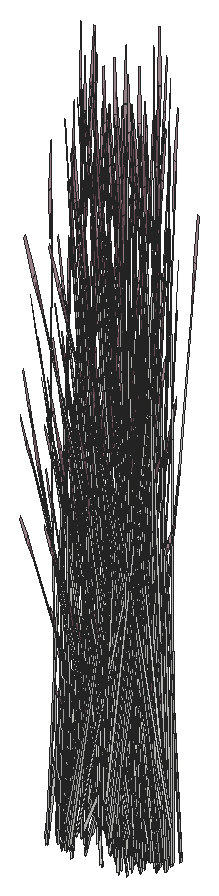
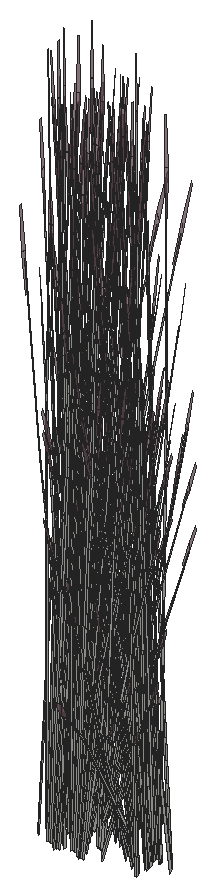
# SketchUp Ruby script. Lengths in inches.
U = 1.inch
M = Sketchup.active_model
def pt(a) = Geom::Point3d.new(a.map { |v| v * U })
def face(e, loops, mat)
  f = e.add_face(loops[0].map { |a| pt(a) })
  loops[1..].each { |l| e.add_face(l.map { |a| pt(a) }).erase! }
  f.material = f.back_material = mat if mat
  f
end
# faces: each face lists its corners as indices into pts; further lists are holes
def faces(e, pts, list, mat = nil) = list.each { |f| face(e, (f[0].is_a?(Array) ? f : [f]).map { |l| l.map { |i| pts[i] } }, mat) }
# xy, xz, yz: faces in a plane at the given z, y or x. An outline is a flat list of corners, or four numbers for a rectangle; further outlines are holes
def ring(l) = l.size == 4 ? [[l[0], l[1]], [l[2], l[1]], [l[2], l[3]], [l[0], l[3]]] : l.each_slice(2).to_a
def flat(e, list, mat, &to3) = list.each { |f| face(e, (f[0].is_a?(Array) ? f : [f]).map { |l| ring(l).map { |u, v| to3.(u, v) } }, mat) }
def xy(e, z, list, mat = nil) = flat(e, list, mat) { |x, y| [x, y, z] }
def xz(e, y, list, mat = nil) = flat(e, list, mat) { |x, z| [x, y, z] }
def yz(e, x, list, mat = nil) = flat(e, list, mat) { |y, z| [x, y, z] }
def lines(e, pts, list) = list.each { |a, b| e.add_line(pt(pts[a]), pt(pts[b])) }
# prism: a flat outline (further loops are holes) pulled along v
def prism(e, loops, v, mat = nil)
  f = face(e, loops, mat); d = Geom::Vector3d.new(v.map { |x| x * U })
  f.pushpull(f.normal.samedirection?(d) ? d.length : -d.length)
end
def box(e, o, s, mat = nil) = prism(e, [[o, [o[0] + s[0], o[1], o[2]], [o[0] + s[0], o[1] + s[1], o[2]], [o[0], o[1] + s[1], o[2]]]], [0, 0, s[2]], mat)
def at(x, y, z, deg = 0) = Geom::Transformation.translation(pt([x, y, z])) * Geom::Transformation.rotation(ORIGIN, Z_AXIS, deg.degrees)
def axes(o, x, y, z) = Geom::Transformation.new([*x, 0, *y, 0, *z, 0, *pt(o).to_a, 1])
def part(name) = M.definitions.add(name)
# library, detail: a bought-in or finely detailed component or shape, given as its bounding box
def library(name, o, s) = part(name).tap { |d| box(d.entities, o, s) }
def detail(e, o, s) = box(e.add_group.entities, o, s)
def put(e, d, t, mat = nil) = e.add_instance(d, t).tap { |i| i.material = mat if mat }
def group(e, t, mat = nil) = e.add_group.tap { |g| g.transformation = t; g.material = mat if mat }.entities
root = M.entities
M.materials.add("LightPink_Translucent").color = [144, 107, 117]
M.materials["LightPink_Translucent"].alpha = 0.75
c1 = part("blade")
p = [[2.15,0.21,22],[0,0.17,0],[0.09,0.45,0],[2.18,0.31,22],[2.29,0.31,22],[0.38,0.45,0],
  [2.48,0.24,33],[2.49,0.24,33],[2.48,0.22,33]]
faces(c1.entities,p,[[0,1,2,3],[4,5,2,3],[6,3,4,7],[8,0,3,6]])
c2 = part("seeds")
p = [[0.3,-0.1,1.38],[-0.01,-0.03,1.59],[-0.01,-0.03,0.03],[0.14,-0.07,-0.07],[0.29,-0.03,3],[0.15,0.01,3.11]]
faces(c2.entities,p,[[0,1,2,3],[1,0,4,5]],"LightPink_Translucent")
c3 = part("blade with seeds")
put(c3.entities,c1,at(0,0,0))
put(c3.entities,c2,axes([2.4,0.25,30.99],[1.5799,-0.05474,1.17369],[-0.12525,1.92788,0.29478],[-0.07173,-0.02425,1.56792]))
put(root,c3,axes([350.21,661.74,620.36],[-0.29264,0.42323,0.45755],[-0.34767,-0.3736,0.17955],[0.07055,-0.04224,1.58856]))
put(root,c3,axes([350.71,662.41,620.21],[0.24637,0.30123,0],[-0.24637,0.30123,0],[0,0,1.69266]))
put(root,c3,axes([350.71,662.06,620.72],[0.17124,-0.42022,0.44739],[0.35581,0.20224,-0.21531],[0,0.09687,1.43643]))
put(root,c3,axes([350.5625,663.52,620.2],[0.35581,0.20937,0],[-0.17124,0.43505,0],[0,0,1.74954]))
put(root,c3,axes([354.72,661.82,621.875],[0.14639,-0.01056,1.71376],[-0.09712,0.45778,0.13857],[-0.20862,-0.02831,0.73262]))
put(root,c3,axes([350.59,661.96,620.38],[-0.44609,-0.09826,0.49198],[0.09078,-0.55493,0.19306],[0.06519,0.05359,1.70813]))
put(root,c3,axes([350.72,662.2,620.21],[0.39487,0,0],[0,0.48281,0],[0,0,1.78407]))
put(root,c3,axes([350.34,661.67,620.72],[-0.21202,-0.39143,0.44739],[0.32115,-0.27564,-0.21531],[0.06861,0.04843,1.43643]))
put(root,c3,axes([349.96,661.77,620.67],[-0.04113,-0.53214,-0.29095],[0.42835,-0.03218,-0.50002],[0.07543,-0.07088,1.59708]))
put(root,c3,axes([350.86,662.15,620.62],[0.32884,-0.136,0.1448],[0.11516,0.38837,-0.41347],[0,0.08547,1.26744]))
put(root,c3,axes([349.9,660.59,620.03],[0.32928,0.11539,-0.30978],[-0.08291,0.40636,0.30978],[0.06638,-0.04686,1.38974]))
put(root,c3,axes([351.61,662.29,620.48],[0,-0.46636,0.49651],[0.39487,0,0],[0,0.10622,1.57504]))
put(root,c3,axes([355.48,662.15,621.34],[0.10032,-0.06746,1.77064],[0.0346,0.47103,0.13857],[-0.2173,0.0625,0.63284]))
put(root,c3,axes([350.48,661.5625,620.62],[0.06809,-0.4162,0.1448],[0.33266,0.07225,-0.41347],[0.06054,0.04274,1.26744]))
put(root,c3,axes([350.96,660.84,620.48],[-0.33032,-0.23318,0.49651],[0.19744,-0.41812,0],[0.07523,0.05311,1.57504]))
put(root,c3,axes([354.4,662.46,622.72],[-0.05763,0.06055,1.74944],[0.0049,0.44239,-0.27667],[-0.13211,0.05753,0.14031]))
put(root,c3,axes([355.15,661.39,622.98],[-0.35281,-0.01123,-0.71045],[0.0237,-0.47284,0.08574],[-0.14947,-0.0499,1.00501]))
put(root,c3,axes([350.67,663.27,620.18],[0.37054,-0.15823,-0.19198],[0.1302,0.45581,0.00008],[0.0409,-0.01749,1.73897]))
put(root,c3,axes([354.87,661.51,620.59],[0.06891,0.12984,1.43002],[-0.15879,0.35293,-0.30754],[-0.16304,-0.08436,0.61141]))
put(root,c3,axes([354.59,662.21,622.53],[-0.29332,-0.1301,-0.35414],[0.08555,-0.37955,0.4572],[-0.11809,0.0348,0.87481]))
put(root,c3,axes([350.68,661.92,620.21],[0.21202,0.39143,-0.44739],[-0.32115,0.27564,0.21531],[0.06861,0.04843,1.43643]))
put(root,c3,axes([354.79,662.4,622.68],[-0.09562,0.42421,-0.51099],[-0.32782,-0.1454,-0.3958],[-0.13199,0.0389,0.97773]))
put(root,c3,axes([355.04,661.49,622.68],[-0.25628,0.30892,-0.51099],[-0.22444,-0.32634,-0.3958],[-0.13021,-0.047,0.97773]))
put(root,c3,axes([354.62,662.375,619.49],[0.00895,0.0735,1.76342],[-0.18044,0.38382,-0.26939],[-0.12817,-0.01935,0.30037]))
put(root,c3,axes([354.67,660.62,622.71],[0.02617,0.04654,1.77383],[-0.12614,0.41836,-0.16761],[-0.12775,0.00303,0.31391]))
put(root,c3,axes([351.26,661.05,620.03],[0.08291,0.40636,-0.30978],[-0.32928,0.11539,0.30978],[0.06638,0.04686,1.38974]))
put(root,c3,axes([354.65,662.16,622.73],[0.09971,-0.42522,0.48003],[0.32782,0.1454,0.3958],[-0.12892,0.02555,0.9933]))
put(root,c3,axes([354.77,662.04,623.03],[0.17758,0.42229,-0.1216],[-0.31518,0.20752,-0.67495],[-0.13282,0.05572,1.02557]))
put(root,c3,axes([355.17,661.16,623.03],[-0.0189,0.47427,-0.1216],[-0.35781,-0.01296,-0.67495],[-0.13781,-0.03295,1.02557]))
put(root,c3,axes([354.94,661.2,622.53],[-0.20082,-0.29199,-0.35414],[0.2293,-0.2764,0.4572],[-0.1165,-0.04206,0.87481]))
put(root,c3,axes([354.63,662.05,622.73],[-0.12963,-0.31798,0.0643],[0.23638,-0.15564,0.50621],[-0.1042,0.03071,0.77189]))
put(root,c3,axes([350.45,661.7,620.67],[0.35635,-0.30962,-0.29095],[0.23697,0.43749,-0.50002],[0.08792,0.04443,1.59708]))
put(root,c3,axes([351.51,661.64,623.05],[-0.30722,0.06665,0.35414],[-0.08112,-0.381,-0.4572],[0.08804,-0.10234,0.87481]))
put(root,c3,axes([354.46,661.9,620.77],[0.22533,-0.03337,1.1486],[-0.14293,0.29403,0.84392],[-0.11135,-0.04411,0.25299]))
put(root,c3,axes([349.55,661.42,619.59],[-0.3474,0.18671,1.28929],[-0.11057,-0.53572,0.50096],[0.21332,0.00891,1.46642]))
put(root,c3,axes([354.91,661.09,623.09],[0.29147,-0.34417,0.53763],[0.25138,0.3655,0.4433],[-0.13675,-0.06349,1.11249]))
put(root,c3,axes([351.15,660.59,620.375],[0.22066,-0.46731,0],[0.36918,0.26061,-0.51607],[0.08408,0.05936,1.63711]))
put(root,c3,axes([351.23,663.375,623.05],[-0.20082,-0.29199,0.35414],[0.2293,-0.2764,-0.4572],[0.1165,0.04206,0.87481]))
put(root,c3,axes([351.35,660.875,620.02],[0.33032,0.23318,-0.49651],[-0.19744,0.41812,0],[0.07523,0.05311,1.57504]))
put(root,c3,axes([354.9,662.17,623.05],[0.29332,0.1301,0.35414],[-0.08555,0.37955,-0.4572],[-0.11809,0.0348,0.87481]))
put(root,c3,axes([356.84,661.83,621.875],[0.14639,-0.01056,1.71376],[-0.09712,0.45778,0.13857],[-0.20862,-0.02831,0.73262]))
put(root,c3,axes([355.04,661.08,622.73],[0.01777,-0.35463,0.0643],[0.26836,0.00972,0.50621],[-0.1028,-0.03711,0.77189]))
put(root,c3,axes([352.11,663.57,621.93],[-0.06755,-0.39203,-0.03492],[0.31928,-0.09013,-0.15832],[0.06667,0.02485,0.52218]))
put(root,c3,axes([351.56,662.56,623.05],[-0.29332,-0.1301,0.35414],[0.08555,-0.37955,-0.4572],[0.11809,-0.0348,0.87481]))
put(root,c3,axes([355.8,663.04,620.06],[-0.36714,-0.07646,-0.62353],[0.07747,-0.47163,-0.16365],[-0.10956,-0.05715,1.37633]))
put(root,c3,axes([355.23,661.35,623.05],[0.20082,0.29199,0.35414],[-0.2293,0.2764,-0.4572],[-0.1165,-0.04206,0.87481]))
put(root,c3,axes([350.87,661.77,620.06],[0.36714,0.07646,-0.62353],[-0.07747,0.47163,-0.16365],[0.10956,0.05715,1.37633]))
put(root,c3,axes([352.43,662.04,620.26],[-0.21881,-0.29821,-0.06488],[0.23965,-0.27324,-0.29416],[0.0679,-0.01924,0.97024]))
put(root,c3,axes([351.79,661.58,622.73],[0.2423,0.19613,0.0643],[-0.14107,0.2793,0.50621],[0.07768,-0.0903,0.77189]))
put(root,c3,axes([355.32,663.94,620.02],[-0.33032,-0.23318,-0.49651],[0.19744,-0.41812,0],[-0.07523,-0.05311,1.57504]))
put(root,c3,axes([355.52,664.22,620.375],[-0.22066,0.46731,0],[-0.36918,-0.26061,-0.51607],[-0.08408,-0.05936,1.63711]))
put(root,c3,axes([351.72,661.5,622.73],[0.08753,0.42921,0.48003],[-0.34336,0.07449,0.3958],[0.1012,-0.10094,0.9933]))
put(root,c3,axes([351.76,661.42,622.53],[0.30722,-0.06665,-0.35414],[0.08112,0.381,0.4572],[0.08804,-0.10234,0.87481]))
put(root,c3,axes([357.61,662.16,621.34],[0.10032,-0.06746,1.77064],[0.0346,0.47103,0.13857],[-0.2173,0.0625,0.63284]))
put(root,c3,axes([351.82,662.67,622.73],[0.12963,0.31798,0.0643],[-0.23638,0.15564,0.50621],[0.1042,-0.03071,0.77189]))
put(root,c3,axes([351.28,663.56,623.03],[0.0189,-0.47427,-0.1216],[0.35781,0.01296,-0.67495],[0.13781,0.03295,1.02557]))
put(root,c3,axes([354.96,660.7,620.13],[-0.10181,0.3808,-0.03893],[-0.31336,-0.11714,-0.17649],[-0.04758,-0.06228,0.58215]))
put(root,c3,axes([351.68,662.68,623.03],[-0.17758,-0.42229,-0.1216],[0.31518,-0.20752,-0.67495],[0.13282,-0.05572,1.02557]))
put(root,c3,axes([351.8,662.56,622.73],[-0.09971,0.42522,0.48003],[-0.32782,-0.1454,0.3958],[0.12892,-0.02555,0.9933]))
put(root,c3,axes([356.53,662.48,622.72],[-0.05763,0.06055,1.74944],[0.0049,0.44239,-0.27667],[-0.13211,0.05753,0.14031]))
put(root,c3,axes([356.22,663.11,620.67],[-0.35635,0.30962,-0.29095],[-0.23697,-0.43749,-0.50002],[-0.08792,-0.04443,1.59708]))
put(root,c3,axes([357.28,661.41,622.98],[-0.35281,-0.01123,-0.71045],[0.0237,-0.47284,0.08574],[-0.14947,-0.0499,1.00501]))
put(root,c3,axes([355.36,656.51,622.76],[0.11138,-0.07357,1.43002],[0.27499,0.22183,-0.30754],[-0.08185,0.19194,0.61141]))
put(root,c3,axes([357,661.52,620.59],[0.06891,0.12984,1.43002],[-0.15879,0.35293,-0.30754],[-0.16304,-0.08436,0.61141]))
put(root,c3,axes([354.79,662.4375,620.375],[-0.44133,0,0],[0,-0.52122,-0.51607],[0,-0.11871,1.63711]))
put(root,c3,axes([355.41,663.76,620.03],[-0.08291,-0.40636,-0.30978],[0.32928,-0.11539,0.30978],[-0.06638,-0.04686,1.38974]))
put(root,c3,axes([356.71,662.22,622.53],[-0.29332,-0.1301,-0.35414],[0.08555,-0.37955,0.4572],[-0.11809,0.0348,0.87481]))
put(root,c3,axes([351.59,663.28,622.72],[0.07571,-0.00789,1.74944],[0.20767,-0.36231,-0.27667],[0.13467,0.04783,0.14031]))
put(root,c3,axes([351.67,662.32,622.68],[0.09562,-0.42421,-0.51099],[0.32782,0.1454,-0.3958],[0.13199,-0.0389,0.97773]))
put(root,c3,axes([352.49,662.59,620.77],[-0.21807,0.07699,1.1486],[0.10265,-0.31819,0.84392],[0.11568,0.02177,0.25299]))
put(root,c3,axes([356.92,662.42,622.68],[-0.09562,0.42421,-0.51099],[-0.32782,-0.1454,-0.3958],[-0.13199,0.0389,0.97773]))
put(root,c3,axes([355.85,660.84,623.05],[0.05451,0.37564,0.35414],[-0.31161,0.09919,-0.4572],[-0.0837,-0.10765,0.87481]))
put(root,c3,axes([355.14,662.3,620.33],[-0.32829,0.39208,0.30756],[-0.32849,-0.38796,-0.36492],[-0.01146,-0.11134,1.64885]))
put(root,c3,axes([357.16,661.5,622.68],[-0.25628,0.30892,-0.51099],[-0.22444,-0.32634,-0.3958],[-0.13021,-0.047,0.97773]))
put(root,c3,axes([356.75,662.39,619.49],[0.00895,0.0735,1.76342],[-0.18044,0.38382,-0.26939],[-0.12817,-0.01935,0.30037]))
put(root,c3,axes([351.87,662.51,622.53],[0.29332,0.1301,-0.35414],[-0.08555,0.37955,0.4572],[0.11809,-0.0348,0.87481]))
put(root,c3,axes([356.49,663.38,621.33],[0.305,0.18805,1.51261],[-0.29879,0.40513,0.59816],[-0.13384,-0.24012,1.26806]))
put(root,c3,axes([356.8,660.64,622.71],[0.02617,0.04654,1.77383],[-0.12614,0.41836,-0.16761],[-0.12775,0.00303,0.31391]))
put(root,c3,axes([356.62,663.25,620.46],[-0.34464,-0.37536,-0.25192],[0.29,-0.42149,0.5513],[-0.0928,0.04391,1.68216]))
put(root,c3,axes([355.99,662.89,620.21],[-0.21202,-0.39143,-0.44739],[0.32115,-0.27564,0.21531],[-0.06861,-0.04843,1.43643]))
put(root,c3,axes([352.02,662.44,619.98],[-0.22732,0.05597,1.41583],[-0.03618,-0.44548,0.08104],[0.15921,-0.06743,0.80566]))
put(root,c3,axes([352.26,662.15,619.49],[-0.01845,-0.0708,1.76342],[0.12793,-0.41416,-0.26939],[0.12905,-0.00596,0.30037]))
put(root,c3,axes([354.625,656.68,624.88],[0.04004,-0.02816,1.77383],[0.33095,0.18728,-0.16761],[-0.00778,0.15594,0.31391]))
put(root,c3,axes([352.39,663.9375,622.71],[-0.03191,-0.04083,1.77383],[0.06981,-0.43764,-0.16761],[0.12571,-0.02796,0.31391]))
put(root,c3,axes([356.45,663.17,620.21],[-0.38326,0.02879,-0.44739],[-0.03466,-0.47788,0.21531],[-0.06861,0.04843,1.43643]))
put(root,c3,axes([351.07,662.04,621.875],[-0.14639,0.01056,1.71376],[0.09712,-0.45778,0.13857],[0.20862,0.02831,0.73262]))
put(root,c3,axes([356.78,662.18,622.73],[0.09971,-0.42522,0.48003],[0.32782,0.1454,0.3958],[-0.12892,0.02555,0.9933]))
put(root,c3,axes([356.9,662.06,623.03],[0.17758,0.42229,-0.1216],[-0.31518,0.20752,-0.67495],[-0.13282,0.05572,1.02557]))
put(root,c3,axes([357.3,661.18,623.03],[-0.0189,0.47427,-0.1216],[-0.35781,-0.01296,-0.67495],[-0.13781,-0.03295,1.02557]))
put(root,c3,axes([357.07,661.21,622.53],[-0.20082,-0.29199,-0.35414],[0.2293,-0.2764,0.4572],[-0.1165,-0.04206,0.87481]))
put(root,c3,axes([356.76,662.06,622.73],[-0.12963,-0.31798,0.0643],[0.23638,-0.15564,0.50621],[-0.1042,0.03071,0.77189]))
put(root,c3,axes([355.71,663.97,620.48],[0.33032,0.23318,0.49651],[-0.19744,0.41812,0],[-0.07523,-0.05311,1.57504]))
put(root,c3,axes([351.6,662.47,622.98],[0.31014,-0.20596,-0.71045],[0.17284,0.42397,0.08574],[0.14985,-0.04816,1.00501]))
put(root,c3,axes([355.63,655.54,625.51],[-0.00918,0.43138,-0.7886],[-0.38672,-0.02897,0.09517],[-0.04081,0.18275,1.11556]))
put(root,c3,axes([356.02,663.12,620.4375],[0.09355,-0.55261,-0.23429],[0.44354,0.09633,0.51271],[-0.0775,-0.07631,1.5644]))
put(root,c3,axes([356.59,661.91,620.77],[0.22533,-0.03337,1.1486],[-0.14293,0.29403,0.84392],[-0.11135,-0.04411,0.25299]))
put(root,c3,axes([356.1875,663.25,620.62],[-0.06809,0.4162,0.1448],[-0.33266,-0.07225,-0.41347],[-0.06054,-0.04274,1.26744]))
put(root,c3,axes([352.65,662.02,622.72],[0.04898,-0.07104,1.74944],[-0.06269,-0.43574,-0.27667],[0.12289,-0.08262,0.14031]))
put(root,c3,axes([354.89,662.08,620.02],[0,-0.46636,-0.49651],[0.39487,0,0],[0,-0.10622,1.57504]))
put(root,c3,axes([355.0625,662.52,620.48],[0,0.46636,0.49651],[-0.39487,0,0],[0,-0.10622,1.57504]))
put(root,c3,axes([357.04,661.1,623.09],[0.29147,-0.34417,0.53763],[0.25138,0.3655,0.4433],[-0.13675,-0.06349,1.11249]))
put(root,c3,axes([355.51,656.15,623.53],[0.00775,-0.24075,1.54345],[0.34877,0.12716,0.21329],[-0.03022,0.25658,0.72882]))
put(root,c3,axes([352.08,663.1,620.59],[-0.085,-0.1147,1.43002],[0.1106,-0.37943,-0.30754],[0.17198,0.0514,0.61141]))
put(root,c3,axes([355.92,662.625,620.67],[-0.39748,-0.22252,-0.29095],[0.19139,-0.46966,-0.50002],[-0.01249,-0.11531,1.59708]))
put(root,c3,axes([357.05,657.58,622.34],[0.04734,0.04659,1.76342],[0.08027,0.4317,-0.26939],[-0.10492,0.09206,0.30037]))
put(root,c3,axes([357.02,662.18,623.05],[0.29332,0.1301,0.35414],[-0.08555,0.37955,-0.4572],[-0.11809,0.0348,0.87481]))
put(root,c3,axes([357.17,661.1,622.73],[0.01777,-0.35463,0.0643],[0.26836,0.00972,0.50621],[-0.1028,-0.03711,0.77189]))
put(root,c3,axes([357.93,663.06,620.06],[-0.36714,-0.07646,-0.62353],[0.07747,-0.47163,-0.16365],[-0.10956,-0.05715,1.37633]))
put(root,c3,axes([355.0625,662.09,620.03],[0.24637,-0.29097,-0.30978],[0.24637,0.29097,0.30978],[0,-0.09372,1.38974]))
put(root,c3,axes([357.35,661.36,623.05],[0.20082,0.29199,0.35414],[-0.2293,0.2764,-0.4572],[-0.1165,-0.04206,0.87481]))
put(root,c3,axes([356.08,662.85,620.36],[0.44609,0.09826,0.45755],[-0.09078,0.55493,0.17955],[-0.06519,-0.05359,1.58856]))
put(root,c3,axes([357.68,656.43,624.72],[0.06572,-0.16029,1.71376],[0.27569,0.33172,0.13857],[-0.12437,0.20675,0.73262]))
put(root,c3,axes([355.96,662.75,620.72],[-0.17124,0.42022,0.44739],[-0.35581,-0.20224,-0.21531],[0,-0.09687,1.43643]))
put(root,c3,axes([356,655.24,624.04],[-0.00864,-0.17899,1.71376],[0.37441,0.11874,0.13857],[-0.02316,0.25508,0.73262]))
put(root,c3,axes([357.45,663.95,620.02],[-0.33032,-0.23318,-0.49651],[0.19744,-0.41812,0],[-0.07523,-0.05311,1.57504]))
put(root,c3,axes([357.65,664.23,620.375],[-0.22066,0.46731,0],[-0.36918,-0.26061,-0.51607],[-0.08408,-0.05936,1.63711]))
put(root,c3,axes([355.84,663.74,620.47],[0.37926,-0.12378,0.17642],[0.09365,0.46065,0.35086],[-0.03382,-0.06712,1.60407]))
put(root,c3,axes([356.9375,657.26,625.56],[-0.00877,0.09229,1.74944],[0.24897,0.32105,-0.27667],[-0.06518,0.15182,0.14031]))
put(root,c3,axes([356.32,663.8125,620.2],[-0.35581,-0.20937,0],[0.17124,-0.43505,0],[0,0,1.62707]))
put(root,c3,axes([357.09,660.71,620.13],[-0.10181,0.3808,-0.03893],[-0.31336,-0.11714,-0.17649],[-0.04758,-0.06228,0.58215]))
put(root,c3,axes([356.96,663.76,620.47],[0.10196,-0.46348,0.17642],[0.3731,0.13116,0.35086],[-0.06445,0.00226,1.60407]))
put(root,c3,axes([356.7,662.8,620.3],[-0.32829,-0.4014,-0.06131],[0.32849,-0.40164,0],[-0.01146,-0.01402,1.75571]))
put(root,c3,axes([356.79,662.94,620.72],[0.38326,-0.02879,0.44739],[0.03466,0.47788,-0.21531],[-0.06861,0.04843,1.43643]))
put(root,c3,axes([358.35,663.13,620.67],[-0.35635,0.30962,-0.29095],[-0.23697,-0.43749,-0.50002],[-0.08792,-0.04443,1.59708]))
put(root,c3,axes([356.04,662.34,620.36],[0.15345,0.52148,0.45755],[-0.43845,0.18134,0.17955],[0.00536,-0.09582,1.58856]))
put(root,c3,axes([356.92,662.45,620.375],[-0.44133,0,0],[0,-0.52122,-0.51607],[0,-0.11871,1.63711]))
put(root,c3,axes([355.97,662.27,620.21],[0.17124,-0.42022,-0.44739],[0.35581,0.20224,0.21531],[0,-0.09687,1.43643]))
put(root,c3,axes([357.54,663.78,620.03],[-0.08291,-0.40636,-0.30978],[0.32928,-0.11539,0.30978],[-0.06638,-0.04686,1.38974]))
put(root,c3,axes([356.41,663.63,620.2],[-0.11516,-0.40207,0],[0.32884,-0.1408,0],[0,0,1.54371]))
put(root,c3,axes([357.65,658.04,623.4375],[0.11138,-0.07357,1.43002],[0.27499,0.22183,-0.30754],[-0.08185,0.19194,0.61141]))
put(root,c3,axes([357.97,660.86,623.05],[0.05451,0.37564,0.35414],[-0.31161,0.09919,-0.4572],[-0.0837,-0.10765,0.87481]))
put(root,c3,axes([357.26,662.32,620.33],[-0.32829,0.39208,0.30756],[-0.32849,-0.38796,-0.36492],[-0.01146,-0.11134,1.64885]))
put(root,c3,axes([358.61,663.4,621.33],[0.305,0.18805,1.51261],[-0.29879,0.40513,0.59816],[-0.13384,-0.24012,1.26806]))
put(root,c3,axes([357.76,657.23,625.58],[-0.25132,-0.3182,0.48003],[0.2669,-0.27442,0.3958],[-0.04636,0.14929,0.9933]))
put(root,c3,axes([358.75,663.27,620.46],[-0.34464,-0.37536,-0.25192],[0.29,-0.42149,0.5513],[-0.0928,0.04391,1.68216]))
put(root,c3,axes([358.12,662.91,620.21],[-0.21202,-0.39143,-0.44739],[0.32115,-0.27564,0.21531],[-0.06861,-0.04843,1.43643]))
put(root,c3,axes([357.55,662.58,620.47],[-0.2773,-0.3397,0.17642],[0.27945,-0.32949,0.35086],[-0.03063,0.06937,1.60407]))
put(root,c3,axes([356.59,662.38,620.21],[0,-0.53961,0],[0.44133,0,0],[0,0,1.79456]))
put(root,c3,axes([357.67,657.2,625.58],[-0.29004,-0.02173,0.0643],[0.00795,-0.32812,0.50621],[-0.03035,0.12569,0.77189]))
put(root,c3,axes([356.18,662.48,620.43],[0.39767,0.22603,0.24065],[-0.19139,0.46966,0.50002],[0,-0.10827,1.60543]))
put(root,c3,axes([356.8125,662.6,620.29],[0,0.53934,-0.05637],[-0.44133,0,0],[0,0.01695,1.79368]))
put(root,c3,axes([356.05,662.17,620.72],[-0.38326,0.02879,0.44739],[-0.03466,-0.47788,-0.21531],[0.06861,-0.04843,1.43643]))
put(root,c3,axes([357.76,657.33,625.37],[-0.23881,0.24554,-0.35414],[-0.22606,-0.28036,0.4572],[-0.0344,0.14245,0.87481]))
put(root,c3,axes([358.57,663.1875,620.21],[-0.38326,0.02879,-0.44739],[-0.03466,-0.47788,0.21531],[-0.06861,0.04843,1.43643]))
put(root,c3,axes([355.87,661.35,620.47],[-0.10196,0.46348,0.17642],[-0.3731,-0.13116,0.35086],[0.06445,-0.00226,1.60407]))
put(root,c3,axes([356.08,656.87,624.88],[0.04474,0.0751,1.74944],[0.36104,0.0295,-0.27667],[0.03631,0.16562,0.14031]))
put(root,c3,axes([356.91,658.2,625.55],[0.04004,-0.02816,1.77383],[0.33095,0.18728,-0.16761],[-0.00778,0.15594,0.31391]))
put(root,c3,axes([357.84,663.99,620.48],[0.33032,0.23318,0.49651],[-0.19744,0.41812,0],[-0.07523,-0.05311,1.57504]))
put(root,c3,axes([358.15,663.13,620.4375],[0.09355,-0.55261,-0.23429],[0.44354,0.09633,0.51271],[-0.0775,-0.07631,1.5644]))
put(root,c3,axes([357,661.37,620.47],[-0.37926,0.12378,0.17642],[-0.09365,-0.46065,0.35086],[0.03382,0.06712,1.60407]))
put(root,c3,axes([358.3125,663.26,620.62],[-0.06809,0.4162,0.1448],[-0.33266,-0.07225,-0.41347],[-0.06054,-0.04274,1.26744]))
put(root,c3,axes([357.92,657.07,626.18],[-0.00918,0.43138,-0.7886],[-0.38672,-0.02897,0.09517],[-0.04081,0.18275,1.11556]))
put(root,c3,axes([357.02,662.1,620.02],[0,-0.46636,-0.49651],[0.39487,0,0],[0,-0.10622,1.57504]))
put(root,c3,axes([357.19,662.53,620.48],[0,0.46636,0.49651],[-0.39487,0,0],[0,-0.10622,1.57504]))
put(root,c3,axes([357.91,658.28,623.61],[-0.00913,-0.2773,1.1486],[0.22824,0.19778,0.84392],[-0.04489,0.13217,0.25299]))
put(root,c3,axes([356.38,662.04,620.36],[-0.29264,0.42323,0.45755],[-0.34767,-0.3736,0.17955],[0.07055,-0.04224,1.58856]))
put(root,c3,axes([356.88,662.71,620.21],[0.24637,0.30123,0],[-0.24637,0.30123,0],[0,0,1.69266]))
put(root,c3,axes([356.875,662.36,620.72],[0.17124,-0.42022,0.44739],[0.35581,0.20224,-0.21531],[0,0.09687,1.43643]))
put(root,c3,axes([356.34,655.91,625.15],[0.16845,0.3792,-0.71045],[-0.34676,0.21133,0.08574],[0.03939,0.18322,1.00501]))
put(root,c3,axes([358.05,662.64,620.67],[-0.39748,-0.22252,-0.29095],[0.19139,-0.46966,-0.50002],[-0.01249,-0.11531,1.59708]))
put(root,c3,axes([356.76,662.26,620.38],[-0.44609,-0.09826,0.49198],[0.09078,-0.55493,0.19306],[0.06519,0.05359,1.70813]))
put(root,c3,axes([357.79,657.68,624.21],[0.00775,-0.24075,1.54345],[0.34877,0.12716,0.21329],[-0.03022,0.25658,0.72882]))
put(root,c3,axes([356.89,662.5,620.21],[0.39487,0,0],[0,0.48281,0],[0,0,1.78407]))
put(root,c3,axes([356.51,661.97,620.72],[-0.21202,-0.39143,0.44739],[0.32115,-0.27564,-0.21531],[0.06861,0.04843,1.43643]))
put(root,c3,axes([356.125,662.07,620.67],[-0.04113,-0.53214,-0.29095],[0.42835,-0.03218,-0.50002],[0.07543,-0.07088,1.59708]))
put(root,c3,axes([357.03,662.46,620.62],[0.32884,-0.136,0.1448],[0.11516,0.38837,-0.41347],[0,0.08547,1.26744]))
put(root,c3,axes([357.19,662.11,620.03],[0.24637,-0.29097,-0.30978],[0.24637,0.29097,0.30978],[0,-0.09372,1.38974]))
put(root,c3,axes([358,657.21,625.85],[0.25266,0.31335,-0.5672],[-0.2669,0.27442,-0.43934],[-0.03844,0.15921,1.08528]))
put(root,c3,axes([358.2,662.87,620.36],[0.44609,0.09826,0.45755],[-0.09078,0.55493,0.17955],[-0.06519,-0.05359,1.58856]))
put(root,c3,axes([356.07,660.89,620.03],[0.32928,0.11539,-0.30978],[-0.08291,0.40636,0.30978],[0.06638,-0.04686,1.38974]))
put(root,c3,axes([358.09,662.77,620.72],[-0.17124,0.42022,0.44739],[-0.35581,-0.20224,-0.21531],[0,-0.09687,1.43643]))
put(root,c3,axes([357.73,657.05,626.24],[0.3879,0.02311,-0.13498],[-0.0106,0.43749,-0.74919],[-0.02694,0.1685,1.13838]))
put(root,c3,axes([357.72,657.68,623.67],[0.32063,-0.08258,0.06507],[0.07371,0.33271,-0.86304],[-0.02033,0.16842,0.7736]))
put(root,c3,axes([357.78,662.59,620.48],[0,-0.46636,0.49651],[0.39487,0,0],[0,0.10622,1.57504]))
put(root,c3,axes([355.99,660.7,620.02],[0.33032,-0.23318,-0.49651],[0.19744,0.41812,0],[0.07523,-0.05311,1.57504]))
put(root,c3,axes([361.18,659.64,626.56],[0.12246,-0.09864,1.71376],[0.1031,0.45582,0.13857],[-0.19225,0.10302,0.73262]))
put(root,c3,axes([356.65,661.86,620.62],[0.06809,-0.4162,0.1448],[0.33266,0.07225,-0.41347],[0.06054,0.04274,1.26744]))
put(root,c3,axes([357.96,663.75,620.47],[0.37926,-0.12378,0.17642],[0.09365,0.46065,0.35086],[-0.03382,-0.06712,1.60407]))
put(root,c3,axes([358.28,656.76,624.72],[-0.00864,-0.17899,1.71376],[0.37441,0.11874,0.13857],[-0.02316,0.25508,0.73262]))
put(root,c3,axes([360.8,660.42,625.27],[0.12266,0.03828,1.43002],[0.07906,0.39104,-0.30754],[-0.16661,0.0732,0.61141]))
put(root,c3,axes([358.45,663.83,620.2],[-0.35581,-0.20937,0],[0.17124,-0.43505,0],[0,0,1.62707]))
put(root,c3,axes([357.125,661.14,620.48],[-0.33032,-0.23318,0.49651],[0.19744,-0.41812,0],[0.07523,0.05311,1.57504]))
put(root,c3,axes([361.88,659.17,626.02],[0.10032,-0.06746,1.77064],[0.0346,0.47103,0.13857],[-0.2173,0.0625,0.63284]))
put(root,c3,axes([356.84,663.57,620.18],[0.37054,-0.15823,-0.19198],[0.1302,0.45581,0.00008],[0.0409,-0.01749,1.73897]))
put(root,c3,axes([359.09,663.78,620.47],[0.10196,-0.46348,0.17642],[0.3731,0.13116,0.35086],[-0.06445,0.00226,1.60407]))
put(root,c3,axes([358.83,662.82,620.3],[-0.32829,-0.4014,-0.06131],[0.32849,-0.40164,0],[-0.01146,-0.01402,1.75571]))
put(root,c3,axes([358.91,662.96,620.72],[0.38326,-0.02879,0.44739],[0.03466,0.47788,-0.21531],[-0.06861,0.04843,1.43643]))
put(root,c3,axes([356.84,662.22,620.21],[0.21202,0.39143,-0.44739],[-0.32115,0.27564,0.21531],[0.06861,0.04843,1.43643]))
put(root,c3,axes([360.8,659.48,627.4],[-0.05763,0.06055,1.74944],[0.0049,0.44239,-0.27667],[-0.13211,0.05753,0.14031]))
put(root,c3,axes([358.17,662.36,620.36],[0.15345,0.52148,0.45755],[-0.43845,0.18134,0.17955],[0.00536,-0.09582,1.58856]))
put(root,c3,axes([358.1,662.29,620.21],[0.17124,-0.42022,-0.44739],[0.35581,0.20224,0.21531],[0,-0.09687,1.43643]))
put(root,c3,axes([358.53,663.64,620.2],[-0.11516,-0.40207,0],[0.32884,-0.1408,0],[0,0,1.54371]))
put(root,c3,axes([360.99,659.23,627.21],[-0.29332,-0.1301,-0.35414],[0.08555,-0.37955,0.4572],[-0.11809,0.0348,0.87481]))
put(root,c3,axes([358.55,657.68,625.91],[-0.34777,-0.12192,0.53283],[0.11892,-0.40083,0.43934],[0.0209,0.15763,1.10256]))
put(root,c3,axes([356.38,661.66,620.06],[0.23773,-0.35053,-0.62353],[0.29532,0.31785,-0.16365],[0.09526,-0.08744,1.37633]))
